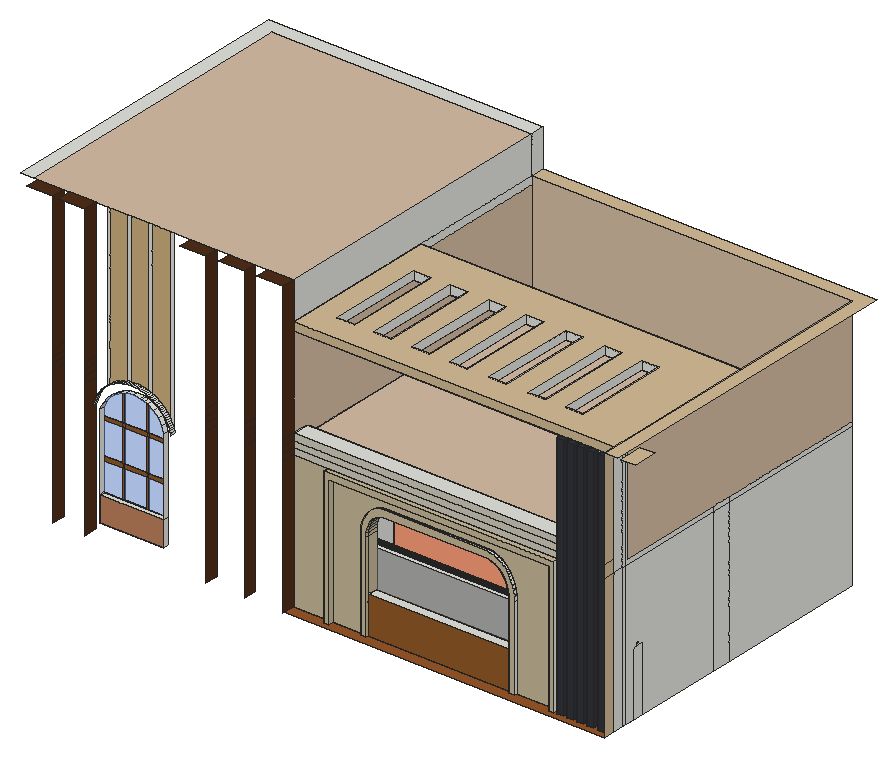
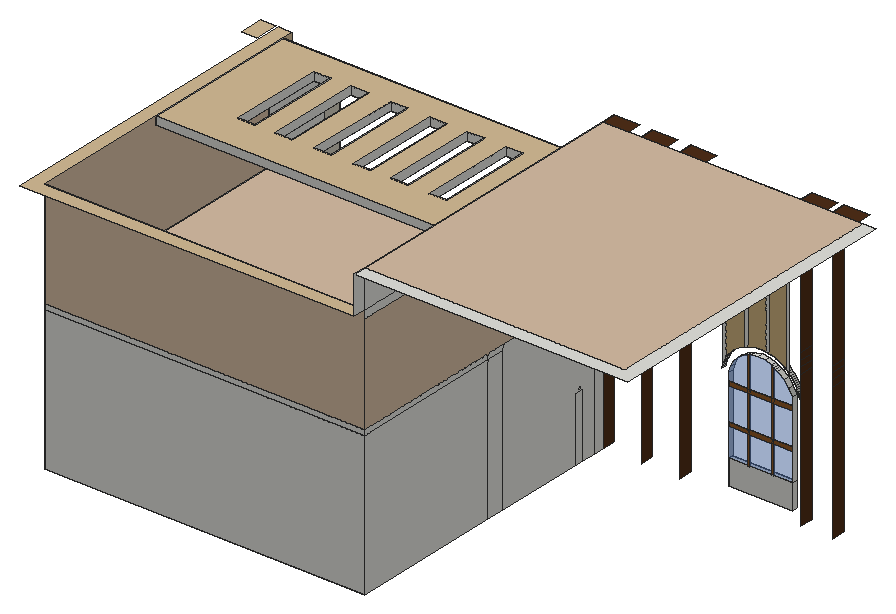
# SketchUp Ruby script. Lengths in inches.
U = 1.inch
M = Sketchup.active_model
def pt(a) = Geom::Point3d.new(a.map { |v| v * U })
def face(e, loops, mat)
  f = e.add_face(loops[0].map { |a| pt(a) })
  loops[1..].each { |l| e.add_face(l.map { |a| pt(a) }).erase! }
  f.material = f.back_material = mat if mat
  f
end
# faces: each face lists its corners as indices into pts; further lists are holes
def faces(e, pts, list, mat = nil) = list.each { |f| face(e, (f[0].is_a?(Array) ? f : [f]).map { |l| l.map { |i| pts[i] } }, mat) }
# xy, xz, yz: faces in a plane at the given z, y or x. An outline is a flat list of corners, or four numbers for a rectangle; further outlines are holes
def ring(l) = l.size == 4 ? [[l[0], l[1]], [l[2], l[1]], [l[2], l[3]], [l[0], l[3]]] : l.each_slice(2).to_a
def flat(e, list, mat, &to3) = list.each { |f| face(e, (f[0].is_a?(Array) ? f : [f]).map { |l| ring(l).map { |u, v| to3.(u, v) } }, mat) }
def xy(e, z, list, mat = nil) = flat(e, list, mat) { |x, y| [x, y, z] }
def xz(e, y, list, mat = nil) = flat(e, list, mat) { |x, z| [x, y, z] }
def yz(e, x, list, mat = nil) = flat(e, list, mat) { |y, z| [x, y, z] }
def lines(e, pts, list) = list.each { |a, b| e.add_line(pt(pts[a]), pt(pts[b])) }
# prism: a flat outline (further loops are holes) pulled along v
def prism(e, loops, v, mat = nil)
  f = face(e, loops, mat); d = Geom::Vector3d.new(v.map { |x| x * U })
  f.pushpull(f.normal.samedirection?(d) ? d.length : -d.length)
end
def box(e, o, s, mat = nil) = prism(e, [[o, [o[0] + s[0], o[1], o[2]], [o[0] + s[0], o[1] + s[1], o[2]], [o[0], o[1] + s[1], o[2]]]], [0, 0, s[2]], mat)
def at(x, y, z, deg = 0) = Geom::Transformation.translation(pt([x, y, z])) * Geom::Transformation.rotation(ORIGIN, Z_AXIS, deg.degrees)
def axes(o, x, y, z) = Geom::Transformation.new([*x, 0, *y, 0, *z, 0, *pt(o).to_a, 1])
def part(name) = M.definitions.add(name)
# library, detail: a bought-in or finely detailed component or shape, given as its bounding box
def library(name, o, s) = part(name).tap { |d| box(d.entities, o, s) }
def detail(e, o, s) = box(e.add_group.entities, o, s)
def put(e, d, t, mat = nil) = e.add_instance(d, t).tap { |i| i.material = mat if mat }
def group(e, t, mat = nil) = e.add_group.tap { |g| g.transformation = t; g.material = mat if mat }.entities
root = M.entities
M.materials.add("[0026_LightSalmon]").color = [255, 160, 122]
M.materials.add("[Blinds Cloth Horizontal]").color = [192, 163, 85]
M.materials.add("[Formica Beige]").color = [211, 187, 149]
M.materials.add("[Formica Graystone]").color = [209, 204, 189]
M.materials.add("[Formica Laminate Dark]").color = [50, 53, 60]
M.materials.add("[Formica Laminate Light]").color = [213, 189, 164]
M.materials.add("[Quartz Light Brown]").color = [199, 184, 152]
M.materials.add("[Translucent Glass Blue]").color = [100, 149, 237]
M.materials["[Translucent Glass Blue]"].alpha = 0.5
M.materials.add("[Translucent Glass Gray]").color = [128, 128, 128]
M.materials["[Translucent Glass Gray]"].alpha = 0.5
M.materials.add("[Wood Board Cork]").color = [215, 201, 115]
M.materials.add("[Wood Cherry Original]").color = [152, 86, 42]
M.materials.add("[Wood Floor Light]").color = [204, 176, 127]
M.materials.add("[Wood Floor Parquet]").color = [145, 89, 39]
M.materials.add("[Wood Lumber ButtJoined]").color = [164, 152, 112]
M.materials.add("[Wood Veneer 01]").color = [79, 46, 24]
M.materials.add("[Wood Veneer 02]").color = [190, 128, 91]
xy(root,384.375,[[396.28,197.36,402.37,203.79],[656.81,197.36,662.9,203.79],[665.86,197.92,673.64,203.79],[677.3,197.92,685.08,203.79],[688.86,197.92,696.64,203.79],
  [700.67,197.92,708.46,203.79],[713.49,197.92,721.27,203.79],[436.36,200.73,443.05,203.79],[608.17,200.73,614.86,203.79],[356.6875,203.79,443.05,215.49],
  [443.05,203.79,608.17,215.49],[608.17,203.79,727.17,215.49],[356.6875,215.49,727.17,232.67],[356.6875,232.67,727.17,244.16],[356.6875,244.16,727.17,348.07],
  [356.6875,348.07,727.17,370.07],[356.6875,370.07,727.17,548.03]])
xy(root,384.375,[[356.6875,190.11,727.17,190.11,727.17,203.79,721.27,203.79,721.27,197.92,713.49,197.92,713.49,203.79,708.46,203.79,708.46,197.92,700.67,197.92,700.67,203.79,696.64,203.79,696.64,197.92,688.86,197.92,688.86,203.79,685.08,203.79,685.08,197.92,677.3,197.92,677.3,203.79,673.64,203.79,673.64,197.92,665.86,197.92,665.86,203.79,662.9,203.79,662.9,197.36,656.81,197.36,656.81,203.79,614.86,203.79,614.86,200.73,608.17,200.73,608.17,203.79,443.05,203.79,443.05,200.73,436.36,200.73,436.36,203.79,402.37,203.79,402.37,197.36,396.28,197.36,396.28,203.79,356.6875,203.79]],"[Wood Cherry Original]")
xy(root,397.07,[[137.48,197.92,211.51,203.79]])
xy(root,425.68,[[137.48,197.92,211.51,203.79]])
xy(root,427.25,[[443.05,203.79,608.17,215.49]])
xy(root,436.87,[[372.34,348.07,438.53,355.26]])
xy(root,458.75,[[356.6875,232.67,727.17,244.16]])
xy(root,514.98,[[463.23,200.73,582.11,203.79],[463.23,203.79,582.11,215.49]])
xy(root,519.81,[[372.34,348.07,438.53,355.26]])
xy(root,522.81,[[462.98,200.73,582.35,203.79]],"[Quartz Light Brown]")
xy(root,534.39,[[402.37,197.36,656.81,203.79]])
xy(root,541.34,[[396.28,197.36,662.9,203.79]],"[Quartz Light Brown]")
xy(root,549,[[356.6875,348.07,727.17,370.07],[356.6875,370.07,727.17,548.03]])
xy(root,555.125,[[356.6875,223.7,727.17,548.03]],"[Formica Laminate Light]")
xy(root,563.875,[[356.6875,203.79,662.9,223.7]])
xy(root,670.25,[[[356.6875,203.79,356.6875,387.77,727.17,387.77,727.17,223.7,662.9,223.7,662.9,203.79],[382.94,233.99,402.82,344.43],[425.38,233.99,445.26,344.43],[469.76,233.99,489.63,344.43],[513.32,233.99,533.19,344.43],[558.69,233.99,578.57,344.43],[604.07,233.99,623.94,344.43],[647.13,233.99,667.01,344.43]]],"[Formica Beige]")
xy(root,670.25,[[665.86,197.92,673.64,203.79],[677.3,197.92,685.08,203.79],[688.86,197.92,696.64,203.79],[700.67,197.92,708.46,203.79],[713.49,197.92,721.27,203.79]],"[Formica Laminate Dark]")
xy(root,679.64,[[727.17,190.11,742.93,190.11,742.93,563.79,356.6875,563.79,356.6875,548.03,727.17,548.03],[746.31,190.11,763.24,218.11],[[356.6875,203.79,727.17,387.77],[382.94,233.99,402.82,344.43],[425.38,233.99,445.26,344.43],[469.76,233.99,489.63,344.43],[513.32,233.99,533.19,344.43],[558.69,233.99,578.57,344.43],[604.07,233.99,623.94,344.43],[647.13,233.99,667.01,344.43]]],"[Formica Beige]")
xy(root,723.1875,[[40.4375,203.79,56.2,203.79,56.2,548.03,356.6875,548.03,356.6875,563.79,40.4375,563.79]])
xy(root,723.1875,[[56.2,203.79,356.6875,548.03]],"[Formica Laminate Light]")
xy(root,723.1875,[[61.07,188.11,91,203.79],[98.07,188.11,128,203.79],[238.01,188.11,267.9375,203.79],[282.39,188.11,312.3125,203.79],[326.76,188.11,356.6875,203.79]],"[Wood Veneer 01]")
xz(root,197.36,[[396.28,384.375,402.37,384.375,402.37,534.39,656.81,534.39,656.81,384.375,662.9,384.375,662.9,541.34,396.28,541.34]],"[Quartz Light Brown]")
xz(root,197.92,[[665.86,384.375,673.64,670.25],[677.3,384.375,685.08,670.25],[688.86,384.375,696.64,670.25],[700.67,384.375,708.46,670.25],[713.49,384.375,721.27,670.25]],"[Formica Laminate Dark]")
xz(root,197.92,[[137.48,397.07,211.51,425.68]],"[Wood Veneer 02]")
xz(root,200.73,[[436.36,384.375,443.05,384.375,443.05,488.3125,443.24,492.08,443.78,495.56,444.66,498.89,445.86,502.03,447.36,504.91,449.12,507.5,451.1,509.73,453.26,511.6,455.57,513.0625,457.99,514.12,460.47,514.75,463.23,514.98,582.11,514.98,585.64,514.6875,588.875,513.86,592.02,512.48,595.02,510.58,597.82,508.17,600.38,505.28,602.65,501.95,604.57,498.24,606.12,494.22,607.25,489.94,607.93,485.5,608.17,480.74,608.17,384.375,614.86,384.375,614.86,480.97,614.58,486.43,613.75,491.8,612.39,496.98,610.51,501.89,608.14,506.4375,605.34,510.55,602.14,514.16,598.61,517.2,594.79,519.625,590.77,521.38,586.6,522.45,582.35,522.81,462.98,522.81,459.51,522.51,456.09,521.64,452.8,520.2,449.67,518.22,446.78,515.73,444.16,512.77,441.86,509.4,439.93,505.68,438.39,501.66,437.27,497.41,436.59,493.02,436.36,488.54]],"[Quartz Light Brown]")
xz(root,203.79,[[396.28,384.375,396.28,541.34,662.9,541.34,662.9,384.375,656.81,384.375,656.81,534.39,402.37,534.39,402.37,384.375],[436.36,384.375,436.36,488.54,436.59,493.02,437.27,497.41,438.39,501.66,439.93,505.68,441.86,509.4,444.16,512.77,446.78,515.73,449.67,518.22,452.8,520.2,456.09,521.64,459.51,522.51,462.98,522.81,582.35,522.81,586.6,522.45,590.77,521.38,594.79,519.625,598.61,517.2,602.14,514.16,605.34,510.55,608.14,506.4375,610.51,501.89,612.39,496.98,613.75,491.8,614.58,486.43,614.86,480.97,614.86,384.375,608.17,384.375,608.17,480.74,607.93,485.5,607.25,489.94,606.12,494.22,604.57,498.24,602.65,501.95,600.38,505.28,597.82,508.17,595.02,510.58,592.02,512.48,588.875,513.86,585.64,514.6875,582.11,514.98,463.23,514.98,460.47,514.75,457.99,514.12,455.57,513.0625,453.26,511.6,451.1,509.73,449.12,507.5,447.36,504.91,445.86,502.03,444.66,498.89,443.78,495.56,443.24,492.08,443.05,488.3125,443.05,384.375],[665.86,384.375,673.64,670.25],[673.64,384.375,677.3,670.25],[677.3,384.375,685.08,670.25],
  [685.08,384.375,688.86,670.25],[688.86,384.375,696.64,670.25],[696.64,384.375,700.67,670.25],[700.67,384.375,708.46,670.25],[708.46,384.375,713.49,670.25],
  [713.49,384.375,721.27,670.25],[721.27,384.375,727.17,670.25],[137.48,397.07,211.51,425.68],[218.4,519.9,218.4,723.1875,215.12,723.1875,215.12,527.48,216.07,525.64,216.93,523.77,217.71,521.85],[141.18,537.45,142.64,538.91,144.17,540.3,144.17,723.1875,141.18,723.1875],
  [192.6,547.93,192.6,723.1875,188.73,723.1875,188.73,549.38,190.68,548.7],[164.25,550.47,166.27,550.89,168.3125,551.21,168.3125,723.1875,164.25,723.1875]])
xz(root,203.79,[[356.6875,670.25,727.17,679.64]],"[Formica Beige]")
xz(root,203.79,[[662.9,384.375,665.86,670.25],[356.6875,541.34,662.9,549],[356.6875,549,662.9,556.4375],[356.6875,556.4375,662.9,563.875]],"[Formica Graystone]")
xz(root,203.79,[[356.6875,384.375,396.28,541.34],[402.37,384.375,436.36,384.375,436.36,488.54,436.59,493.02,437.27,497.41,438.39,501.66,439.93,505.68,441.86,509.4,444.16,512.77,446.78,515.73,449.67,518.22,452.8,520.2,456.09,521.64,459.51,522.51,462.98,522.81,582.35,522.81,586.6,522.45,590.77,521.38,594.79,519.625,598.61,517.2,602.14,514.16,605.34,510.55,608.14,506.4375,610.51,501.89,612.39,496.98,613.75,491.8,614.58,486.43,614.86,480.97,614.86,384.375,656.81,384.375,656.81,534.39,402.37,534.39]],"[Quartz Light Brown]")
xz(root,203.79,[[137.48,425.68,158.65,458.55],[161.03,425.68,186.27,458.55],[188.66,425.68,211.51,458.55],[137.48,463.21,158.65,500.75],[161.03,463.21,186.27,500.75],
  [188.66,463.21,211.51,500.75],[137.48,505.34,158.65,505.34,158.65,538.17,156.35,536.79,153.96,535.3,146.84,529.54,141.18,522.34,137.48,514.54],[161.03,505.34,186.27,505.34,186.27,541.26,184.83,541.79,176.79,542.85,168.71,542.1,161,539.58,161.03,533.51],[188.66,505.34,211.51,505.34,211.51,514.54,209.09,521.8,204.875,528.73,199.23,534.55,192.4375,538.98,188.66,540.38]],"[Translucent Glass Blue]")
xz(root,203.79,[[215.12,527.48,215.12,723.1875,192.6,723.1875,192.6,547.93,194.48,547.08,196.33,546.15,198.125,545.13,199.88,544.04,201.58,542.87,203.23,541.62,204.82,540.3,206.35,538.91,207.8125,537.45,209.21,535.93,210.54,534.35,211.8,532.71,212.99,531.02,214.09,529.27],[144.17,540.3,145.76,541.62,147.41,542.87,149.11,544.04,150.87,545.13,152.66,546.15,154.51,547.08,156.39,547.93,158.3125,548.7,160.26,549.38,162.24,549.97,164.25,550.47,164.25,723.1875,144.17,723.1875],[188.73,549.38,188.73,723.1875,168.3125,723.1875,168.3125,551.21,170.37,551.44,172.43,551.58,174.5,551.625,176.5625,551.58,178.625,551.44,180.68,551.21,182.72,550.89,184.74,550.47,186.75,549.97]],"[Wood Floor Light]")
xz(root,203.79,[[443.05,384.375,608.17,427.25],[158.65,425.68,161.03,458.55],[186.27,425.68,188.66,458.55],[137.48,458.55,158.65,463.21],[158.65,458.55,161.03,463.21],
  [161.03,458.55,186.27,463.21],[186.27,458.55,188.66,463.21],[188.66,458.55,211.51,463.21],[158.65,463.21,161.03,500.75],[186.27,463.21,188.66,500.75],
  [137.48,500.75,158.65,505.34],[158.65,500.75,161.03,505.34],[161.03,500.75,186.27,505.34],[186.27,500.75,188.66,505.34],[188.66,500.75,211.51,505.34],
  [158.65,505.34,161.03,505.34,161.03,533.51,161,539.58,158.65,538.17],[186.27,505.34,188.66,505.34,188.66,540.38,186.27,541.26]],"[Wood Floor Parquet]")
xz(root,215.49,[[443.05,384.375,608.17,427.25]])
xz(root,223.7,[[356.6875,555.125,662.9,563.875],[662.9,555.125,727.17,670.25]])
xz(root,232.67,[[356.6875,384.375,727.17,458.75]],"[Translucent Glass Gray]")
xz(root,233.99,[[382.94,670.25,402.82,679.64],[425.38,670.25,445.26,679.64],[469.76,670.25,489.63,679.64],[513.32,670.25,533.19,679.64],[558.69,670.25,578.57,679.64],
  [604.07,670.25,623.94,679.64],[647.13,670.25,667.01,679.64]])
xz(root,244.16,[[356.6875,384.375,727.17,458.75]])
xz(root,344.43,[[382.94,670.25,402.82,679.64],[425.38,670.25,445.26,679.64],[469.76,670.25,489.63,679.64],[513.32,670.25,533.19,679.64],[558.69,670.25,578.57,679.64],
  [604.07,670.25,623.94,679.64],[647.13,670.25,667.01,679.64]])
xz(root,348.07,[[[356.6875,384.375,630.64,384.375,630.64,526.3125,701.89,526.3125,701.89,384.375,727.17,384.375,727.17,549,356.6875,549],[473.14,434.83,573.76,527.39],[372.34,436.87,438.53,519.81]]],"[0026_LightSalmon]")
xz(root,348.07,[[478.96,440.65,520.59,521.5625],[526.38,440.65,567.9375,521.5625]],"[Blinds Cloth Horizontal]")
xz(root,348.07,[[636.07,469.29,691.81,520.89,687.15,520.89,663.14,499.1,661.61,497.71,636.07,474.53],[661.61,497.71,663.14,499.1,653.11,520.89,649.25,520.89]],"[Wood Board Cork]")
xz(root,348.07,[[[636.07,389.8,696.47,389.8,696.47,520.89,691.81,520.89,636.07,469.29],[640.62,439.3125,644.62,462.125]],[636.07,474.53,661.61,497.71,649.25,520.89,636.07,520.89],[663.14,499.1,687.15,520.89,653.11,520.89]],"[Wood Floor Light]")
xz(root,348.07,[[[630.64,384.375,701.89,526.3125],[636.07,389.8,696.47,520.89]],[[473.14,434.83,573.76,527.39],[478.96,440.65,567.9375,521.5625]],[520.59,440.65,526.38,521.5625]],"[Wood Floor Parquet]")
xz(root,348.07,[[640.62,439.3125,644.62,462.125]],"[Wood Lumber ButtJoined]")
xz(root,355.26,[[377.09,441.62,401.32,515.0625],[406.17,441.62,433.78,515.0625]],"[Blinds Cloth Horizontal]")
xz(root,355.26,[[[372.34,436.87,438.53,519.81],[377.09,441.62,433.78,515.0625]],[401.32,441.62,406.17,515.0625]],"[Wood Floor Parquet]")
xz(root,370.07,[[356.6875,384.375,727.17,549]])
xz(root,387.77,[[356.6875,670.25,727.17,679.64]])
xz(root,548.03,[[356.6875,384.375,727.17,549],[356.6875,549,727.17,555.125]])
xz(root,548.03,[[356.6875,555.125,727.17,679.64]],"[Formica Laminate Light]")
yz(root,91,[[188.11,384.375,203.79,541.34],[188.11,541.34,203.79,549],[188.11,549,203.79,556.4375],[188.11,556.4375,203.79,563.875],[188.11,563.875,203.79,723.1875]],"[Wood Veneer 01]")
yz(root,128,[[188.11,384.375,203.79,541.34],[188.11,541.34,203.79,549],[188.11,549,203.79,556.4375],[188.11,556.4375,203.79,563.875],[188.11,563.875,203.79,723.1875]],"[Wood Veneer 01]")
yz(root,137.48,[[197.92,397.07,203.79,425.68],[197.92,425.68,203.79,514.54]])
yz(root,211.51,[[197.92,397.07,203.79,425.68],[197.92,425.68,203.79,514.54]])
yz(root,267.9375,[[188.11,384.375,203.79,541.34],[188.11,541.34,203.79,549],[188.11,549,203.79,556.4375],[188.11,556.4375,203.79,563.875],[188.11,563.875,203.79,723.1875]],"[Wood Veneer 01]")
yz(root,312.3125,[[188.11,384.375,203.79,541.34],[188.11,541.34,203.79,549],[188.11,549,203.79,556.4375],[188.11,556.4375,203.79,563.875],[188.11,563.875,203.79,723.1875]],"[Wood Veneer 01]")
yz(root,356.6875,[[203.79,384.375,215.49,563.875],[[215.49,384.375,232.67,384.375,232.67,458.75,244.16,458.75,244.16,384.375,348.07,384.375,348.07,555.125,223.7,555.125,223.7,563.875,215.49,563.875],[237.55,459.44,236.99,459.51,236.46,459.73,236.01,460.08,235.66,460.53,235.44,461.06,235.37,461.62,235.44,462.1875,235.66,462.72,236.01,463.17,236.46,463.52,236.99,463.74,237.55,463.81,238.12,463.74,238.65,463.52,239.1,463.17,239.45,462.72,239.67,462.1875,239.74,461.62,239.67,461.06,239.45,460.53,239.1,460.08,238.65,459.73,238.12,459.51]],[232.67,384.375,244.16,458.75],[348.07,384.375,370.07,549],[370.07,384.375,548.03,549],
  [237.55,459.44,236.99,459.51,236.46,459.73,236.01,460.08,235.66,460.53,235.44,461.06,235.37,461.62,235.44,462.1875,235.66,462.72,236.01,463.17,236.46,463.52,236.99,463.74,237.55,463.81,238.12,463.74,238.65,463.52,239.1,463.17,239.45,462.72,239.67,462.1875,239.74,461.62,239.67,461.06,239.45,460.53,239.1,460.08,238.65,459.73,238.12,459.51],[348.07,549,370.07,555.125],[370.07,549,548.03,555.125],[203.79,670.25,387.77,679.64],[387.77,670.25,548.03,679.64],
  [203.79,679.64,548.03,723.1875],[548.03,679.64,563.79,723.1875]])
yz(root,356.6875,[[223.7,555.125,548.03,555.125,548.03,670.25,203.79,670.25,203.79,563.875,223.7,563.875]],"[Formica Laminate Light]")
yz(root,356.6875,[[188.11,384.375,203.79,541.34],[188.11,541.34,203.79,549],[188.11,549,203.79,556.4375],[188.11,556.4375,203.79,563.875],[188.11,563.875,203.79,723.1875]],"[Wood Veneer 01]")
yz(root,372.34,[[348.07,436.87,355.26,519.81]])
yz(root,382.94,[[233.99,670.25,344.43,679.64]])
yz(root,396.28,[[197.36,384.375,203.79,541.34]],"[Quartz Light Brown]")
yz(root,402.37,[[197.36,384.375,203.79,534.39]],"[Quartz Light Brown]")
yz(root,402.82,[[233.99,670.25,344.43,679.64]])
yz(root,425.38,[[233.99,670.25,344.43,679.64]])
yz(root,436.36,[[200.73,384.375,203.79,488.54]],"[Quartz Light Brown]")
yz(root,438.53,[[348.07,436.87,355.26,519.81]])
yz(root,443.05,[[203.79,384.375,215.49,427.25]])
yz(root,443.05,[[200.73,384.375,203.79,488.3125],[203.79,427.25,215.49,488.3125]],"[Quartz Light Brown]")
yz(root,445.26,[[233.99,670.25,344.43,679.64]])
yz(root,469.76,[[233.99,670.25,344.43,679.64]])
yz(root,489.63,[[233.99,670.25,344.43,679.64]])
yz(root,513.32,[[233.99,670.25,344.43,679.64]])
yz(root,533.19,[[233.99,670.25,344.43,679.64]])
yz(root,558.69,[[233.99,670.25,344.43,679.64]])
yz(root,578.57,[[233.99,670.25,344.43,679.64]])
yz(root,604.07,[[233.99,670.25,344.43,679.64]])
yz(root,608.17,[[203.79,384.375,215.49,427.25]])
yz(root,608.17,[[200.73,384.375,203.79,480.74],[203.79,427.25,215.49,480.74]],"[Quartz Light Brown]")
yz(root,614.86,[[200.73,384.375,203.79,480.97]])
yz(root,623.94,[[233.99,670.25,344.43,679.64]])
yz(root,647.13,[[233.99,670.25,344.43,679.64]])
yz(root,656.81,[[197.36,384.375,203.79,534.39]],"[Quartz Light Brown]")
yz(root,662.9,[[197.36,384.375,203.79,541.34]])
yz(root,662.9,[[203.79,563.875,223.7,670.25]],"[Formica Graystone]")
yz(root,665.86,[[197.92,384.375,203.79,670.25]],"[Formica Laminate Dark]")
yz(root,667.01,[[233.99,670.25,344.43,679.64]])
yz(root,673.64,[[197.92,384.375,203.79,670.25]],"[Formica Laminate Dark]")
yz(root,677.3,[[197.92,384.375,203.79,670.25]],"[Formica Laminate Dark]")
yz(root,685.08,[[197.92,384.375,203.79,670.25]],"[Formica Laminate Dark]")
yz(root,688.86,[[197.92,384.375,203.79,670.25]],"[Formica Laminate Dark]")
yz(root,696.64,[[197.92,384.375,203.79,670.25]],"[Formica Laminate Dark]")
yz(root,700.67,[[197.92,384.375,203.79,670.25]],"[Formica Laminate Dark]")
yz(root,708.46,[[197.92,384.375,203.79,670.25]],"[Formica Laminate Dark]")
yz(root,713.49,[[197.92,384.375,203.79,670.25]],"[Formica Laminate Dark]")
yz(root,721.27,[[197.92,384.375,203.79,670.25]],"[Formica Laminate Dark]")
yz(root,727.17,[[203.79,384.375,215.49,549],[215.49,384.375,219.56,549],[[219.56,384.375,219.56,549,348.07,549,348.07,384.375,244.16,384.375,244.16,458.75,232.67,458.75,232.67,384.375],[237.55,459.44,238.12,459.51,238.65,459.73,239.1,460.08,239.45,460.53,239.67,461.06,239.74,461.62,239.67,462.1875,239.45,462.72,239.1,463.17,238.65,463.52,238.12,463.74,237.55,463.81,236.99,463.74,236.46,463.52,236.01,463.17,235.66,462.72,235.44,462.1875,235.37,461.62,235.44,461.06,235.66,460.53,236.01,460.08,236.46,459.73,236.99,459.51]],[232.67,384.375,244.16,458.75],[348.07,384.375,370.07,549],
  [370.07,384.375,548.03,549],[203.79,549,215.49,670.25],[215.49,549,219.56,670.25],[219.56,549,348.07,549,348.07,555.125,223.7,555.125,223.7,670.25,219.56,670.25],[348.07,549,370.07,555.125],
  [370.07,549,548.03,555.125],[203.79,670.25,215.49,679.64],[215.49,670.25,219.56,679.64],[219.56,670.25,387.77,679.64]])
yz(root,727.17,[[190.11,384.375,203.79,549],[190.11,549,203.79,563.875],[190.11,563.875,203.79,679.64]],"[Formica Beige]")
yz(root,727.17,[[223.7,555.125,223.7,670.25,387.77,670.25,387.77,679.64,548.03,679.64,548.03,555.125]],"[Formica Laminate Light]")
p = [[356.6875,236.99,459.51],[356.6875,237.55,459.44],[727.17,237.55,459.44],[727.17,236.99,459.51],[356.6875,238.12,459.51],[727.17,238.12,459.51],
  [356.6875,236.46,459.73],[727.17,236.46,459.73],[356.6875,238.65,459.73],[727.17,238.65,459.73],[356.6875,236.01,460.08],[727.17,236.01,460.08],
  [356.6875,239.1,460.08],[727.17,239.1,460.08],[356.6875,235.66,460.53],[727.17,235.66,460.53],[356.6875,239.45,460.53],[727.17,239.45,460.53],
  [356.6875,235.44,461.06],[727.17,235.44,461.06],[356.6875,239.67,461.06],[727.17,239.67,461.06],[356.6875,235.37,461.62],[727.17,235.37,461.62],
  [356.6875,239.74,461.62],[727.17,239.74,461.62],[356.6875,235.44,462.1875],[727.17,235.44,462.1875],[356.6875,239.67,462.1875],[727.17,239.67,462.1875],
  [356.6875,235.66,462.72],[727.17,235.66,462.72],[356.6875,239.45,462.72],[727.17,239.45,462.72],[356.6875,236.01,463.17],[727.17,236.01,463.17],
  [356.6875,239.1,463.17],[727.17,239.1,463.17],[356.6875,236.46,463.52],[727.17,236.46,463.52],[356.6875,238.65,463.52],[727.17,238.65,463.52],
  [356.6875,236.99,463.74],[727.17,236.99,463.74],[356.6875,238.12,463.74],[727.17,238.12,463.74],[356.6875,237.55,463.81],[727.17,237.55,463.81],
  [607.93,203.79,485.5],[608.17,203.79,480.74],[608.17,200.73,480.74],[607.93,200.73,485.5],[607.93,215.49,485.5],[608.17,215.49,480.74],
  [614.86,203.79,480.97],[614.58,203.79,486.43],[614.58,200.73,486.43],[614.86,200.73,480.97],[607.25,203.79,489.94],[607.25,200.73,489.94],
  [607.25,215.49,489.94],[613.75,203.79,491.8],[613.75,200.73,491.8],[443.05,203.79,488.3125],[443.24,203.79,492.08],[443.24,200.73,492.08],
  [443.05,200.73,488.3125],[443.05,215.49,488.3125],[443.24,215.49,492.08],[436.59,203.79,493.02],[436.36,203.79,488.54],[436.36,200.73,488.54],
  [436.59,200.73,493.02],[606.12,203.79,494.22],[606.12,200.73,494.22],[606.12,215.49,494.22],[612.39,203.79,496.98],[612.39,200.73,496.98],
  [443.78,203.79,495.56],[443.78,200.73,495.56],[443.78,215.49,495.56],[437.27,203.79,497.41],[437.27,200.73,497.41],[604.57,203.79,498.24],
  [604.57,200.73,498.24],[604.57,215.49,498.24],[444.66,203.79,498.89],[444.66,200.73,498.89],[444.66,215.49,498.89],[610.51,203.79,501.89],
  [610.51,200.73,501.89],[438.39,203.79,501.66],[438.39,200.73,501.66],[602.65,203.79,501.95],[602.65,200.73,501.95],[602.65,215.49,501.95],
  [445.86,203.79,502.03],[445.86,200.73,502.03],[445.86,215.49,502.03],[439.93,203.79,505.68],[439.93,200.73,505.68],[608.14,203.79,506.4375],
  [608.14,200.73,506.4375],[447.36,203.79,504.91],[447.36,200.73,504.91],[600.38,203.79,505.28],[600.38,200.73,505.28],[447.36,215.49,504.91],
  [600.38,215.49,505.28],[449.12,203.79,507.5],[449.12,200.73,507.5],[449.12,215.49,507.5],[597.82,203.79,508.17],[597.82,200.73,508.17],
  [597.82,215.49,508.17],[441.86,203.79,509.4],[441.86,200.73,509.4],[605.34,203.79,510.55],[605.34,200.73,510.55],[451.1,203.79,509.73],
  [451.1,200.73,509.73],[451.1,215.49,509.73],[595.02,203.79,510.58],[595.02,200.73,510.58],[595.02,215.49,510.58],[444.16,203.79,512.77],
  [444.16,200.73,512.77],[453.26,203.79,511.6],[453.26,200.73,511.6],[453.26,215.49,511.6],[592.02,203.79,512.48],[592.02,200.73,512.48],
  [602.14,203.79,514.16],[602.14,200.73,514.16],[592.02,215.49,512.48],[455.57,203.79,513.0625],[455.57,200.73,513.0625],[455.57,215.49,513.0625],
  [588.875,203.79,513.86],[588.875,200.73,513.86],[588.875,215.49,513.86],[446.78,203.79,515.73],[446.78,200.73,515.73],[457.99,203.79,514.12],
  [457.99,200.73,514.12],[457.99,215.49,514.12],[585.64,203.79,514.6875],[585.64,200.73,514.6875],[585.64,215.49,514.6875],[460.47,203.79,514.75],
  [460.47,200.73,514.75],[460.47,215.49,514.75],[598.61,203.79,517.2],[598.61,200.73,517.2],[137.48,203.79,514.54],[141.18,203.79,522.34],
  [141.18,197.92,522.34],[137.48,197.92,514.54],[209.09,203.79,521.8],[211.51,203.79,514.54],[211.51,197.92,514.54],[209.09,197.92,521.8],
  [582.11,203.79,514.98],[582.11,200.73,514.98],[582.11,215.49,514.98],[463.23,203.79,514.98],[463.23,200.73,514.98],[463.23,215.49,514.98],
  [449.67,203.79,518.22],[449.67,200.73,518.22],[129.98,203.79,517.93],[129.46,203.79,515.93],[129.46,197.92,515.93],[129.98,197.92,517.93],
  [219.53,203.79,515.93],[219.01,203.79,517.93],[219.01,197.92,517.93],[219.53,197.92,515.93],[594.79,203.79,519.625],[594.79,200.73,519.625],
  [130.59,203.79,519.9],[130.59,197.92,519.9],[218.4,203.79,519.9],[218.4,197.92,519.9],[452.8,203.79,520.2],[452.8,200.73,520.2],
  [590.77,203.79,521.38],[590.77,200.73,521.38],[131.28,203.79,521.85],[131.28,197.92,521.85],[217.71,203.79,521.85],[217.71,197.92,521.85],
  [456.09,203.79,521.64],[456.09,200.73,521.64],[586.6,203.79,522.45],[586.6,200.73,522.45],[459.51,203.79,522.51],[459.51,200.73,522.51],
  [204.875,203.79,528.73],[204.875,197.92,528.73],[132.06,203.79,523.77],[132.06,197.92,523.77],[216.93,203.79,523.77],[216.93,197.92,523.77],
  [146.84,203.79,529.54],[146.84,197.92,529.54],[462.98,203.79,522.81],[462.98,200.73,522.81],[582.35,203.79,522.81],[582.35,200.73,522.81],
  [132.92,203.79,525.64],[132.92,197.92,525.64],[216.07,203.79,525.64],[216.07,197.92,525.64],[133.87,203.79,527.48],[133.87,197.92,527.48],
  [215.12,203.79,527.48],[215.12,197.92,527.48],[134.9,203.79,529.27],[134.9,197.92,529.27],[214.09,203.79,529.27],[214.09,197.92,529.27],
  [199.23,203.79,534.55],[199.23,197.92,534.55],[136,203.79,531.02],[136,197.92,531.02],[212.99,203.79,531.02],[212.99,197.92,531.02],
  [153.96,203.79,535.3],[153.96,197.92,535.3],[137.1875,203.79,532.71],[137.1875,197.92,532.71],[211.8,203.79,532.71],[211.8,197.92,532.71],
  [138.45,203.79,534.35],[138.45,197.92,534.35],[210.54,203.79,534.35],[210.54,197.92,534.35],[139.78,203.79,535.93],[139.78,197.92,535.93],
  [209.21,203.79,535.93],[209.21,197.92,535.93],[192.4375,203.79,538.98],[192.4375,197.92,538.98],[156.35,203.79,536.79],[156.35,197.92,536.79],
  [141.18,203.79,537.45],[141.18,197.92,537.45],[207.8125,203.79,537.45],[207.8125,197.92,537.45],[158.65,203.79,538.17],[158.65,197.92,538.17],
  [142.64,203.79,538.91],[142.64,197.92,538.91],[206.35,203.79,538.91],[206.35,197.92,538.91],[161,203.79,539.58],[161,197.92,539.58],
  [144.17,203.79,540.3],[144.17,197.92,540.3],[204.82,203.79,540.3],[204.82,197.92,540.3],[188.66,203.79,540.38],[188.66,197.92,540.38],
  [168.71,203.79,542.1],[168.71,197.92,542.1],[145.76,203.79,541.62],[145.76,197.92,541.62],[203.23,203.79,541.62],[203.23,197.92,541.62],
  [186.27,203.79,541.26],[186.27,197.92,541.26],[184.83,203.79,541.79],[184.83,197.92,541.79],[147.41,203.79,542.87],[147.41,197.92,542.87],
  [201.58,203.79,542.87],[201.58,197.92,542.87],[176.79,203.79,542.85],[176.79,197.92,542.85],[149.11,203.79,544.04],[149.11,197.92,544.04],
  [199.88,203.79,544.04],[199.88,197.92,544.04],[150.87,203.79,545.13],[150.87,197.92,545.13],[198.125,203.79,545.13],[198.125,197.92,545.13],
  [152.66,203.79,546.15],[152.66,197.92,546.15],[196.33,203.79,546.15],[196.33,197.92,546.15],[154.51,203.79,547.08],[154.51,197.92,547.08],
  [194.48,203.79,547.08],[194.48,197.92,547.08],[156.39,203.79,547.93],[156.39,197.92,547.93],[192.6,203.79,547.93],[192.6,197.92,547.93],
  [158.3125,203.79,548.7],[158.3125,197.92,548.7],[190.68,203.79,548.7],[190.68,197.92,548.7],[160.26,203.79,549.38],[160.26,197.92,549.38],
  [188.73,203.79,549.38],[188.73,197.92,549.38],[162.24,203.79,549.97],[162.24,197.92,549.97],[186.75,203.79,549.97],[186.75,197.92,549.97],
  [164.25,203.79,550.47],[164.25,197.92,550.47],[184.74,203.79,550.47],[184.74,197.92,550.47],[166.27,203.79,550.89],[166.27,197.92,550.89],
  [182.72,203.79,550.89],[182.72,197.92,550.89],[168.3125,203.79,551.21],[168.3125,197.92,551.21],[180.68,203.79,551.21],[180.68,197.92,551.21],
  [170.37,203.79,551.44],[170.37,197.92,551.44],[178.625,203.79,551.44],[178.625,197.92,551.44],[172.43,203.79,551.58],[172.43,197.92,551.58],
  [176.5625,203.79,551.58],[176.5625,197.92,551.58],[174.5,203.79,551.625],[174.5,197.92,551.625]]
faces(root,p,[[0,1,2,3],[1,4,5,2],[6,0,3,7],[4,8,9,5],[10,6,7,11],[8,12,13,9],[14,10,11,15],[12,16,17,13],
  [18,14,15,19],[16,20,21,17],[22,18,19,23],[20,24,25,21],[26,22,23,27],[24,28,29,25],[30,26,27,31],[28,32,33,29],
  [34,30,31,35],[32,36,37,33],[38,34,35,39],[36,40,41,37],[42,38,39,43],[40,44,45,41],[46,42,43,47],[44,46,47,45]],"[Formica Laminate Dark]")
faces(root,p,[[48,49,50,51],[49,48,52,53],[58,48,51,59],[48,58,60,52],[63,64,65,66],[64,63,67,68],[69,70,71,72],[73,58,59,74],
  [58,73,75,60],[64,78,79,65],[78,64,68,80],[81,69,72,82],[83,73,74,84],[73,83,85,75],[78,86,87,79],[86,78,80,88],
  [91,81,82,92],[93,83,84,94],[83,93,95,85],[86,96,97,87],[96,86,88,98],[99,91,92,100],[96,103,104,97],[105,93,94,106],
  [103,96,98,107],[93,105,108,95],[103,109,110,104],[109,103,107,111],[112,105,106,113],[105,112,114,108],[115,99,100,116],[109,119,120,110],
  [119,109,111,121],[122,112,113,123],[112,122,124,114],[125,115,116,126],[119,127,128,120],[127,119,121,129],[130,122,123,131],[122,130,134,124],
  [127,135,136,128],[135,127,129,137],[138,130,131,139],[130,138,140,134],[141,125,126,142],[135,143,144,136],[143,135,137,145],[146,138,139,147],
  [138,146,148,140],[143,149,150,144],[149,143,145,151],[162,146,147,163],[146,162,164,148],[149,165,166,150],[165,149,151,167],[168,141,142,169],
  [184,168,169,185],[192,184,185,193],[196,192,193,197],[206,196,197,207]],"[Quartz Light Brown]")
faces(root,p,[[54,55,56,57],[55,61,62,56],[61,76,77,62],[76,89,90,77],[89,101,102,90],[101,117,118,102],[117,132,133,118],[132,152,153,133],
  [154,155,156,157],[158,159,160,161],[170,171,172,173],[174,175,176,177],[152,178,179,153],[180,170,173,181],[175,182,183,176],[178,186,187,179],
  [188,180,181,189],[182,190,191,183],[186,194,195,187],[198,158,161,199],[200,188,189,201],[190,202,203,191],[155,204,205,156],[194,208,209,195],
  [210,200,201,211],[202,212,213,203],[214,210,211,215],[212,216,217,213],[218,214,215,219],[216,220,221,217],[222,198,199,223],[224,218,219,225],
  [220,226,227,221],[204,228,229,205],[230,224,225,231],[226,232,233,227],[234,230,231,235],[232,236,237,233],[238,234,235,239],[236,240,241,237],
  [242,222,223,243],[228,244,245,229],[246,238,239,247],[240,248,249,241],[244,250,251,245],[252,246,247,253],[248,254,255,249],[250,256,257,251],
  [258,252,253,259],[254,260,261,255],[262,242,243,263],[256,264,265,257],[266,258,259,267],[260,268,269,261],[270,262,263,271],[272,270,271,273],
  [274,266,267,275],[268,276,277,269],[278,272,273,279],[264,278,279,265],[280,274,275,281],[276,282,283,277],[284,280,281,285],[282,286,287,283],
  [288,284,285,289],[286,290,291,287],[292,288,289,293],[290,294,295,291],[296,292,293,297],[294,298,299,295],[300,296,297,301],[298,302,303,299],
  [304,300,301,305],[302,306,307,303],[308,304,305,309],[306,310,311,307],[312,308,309,313],[310,314,315,311],[316,312,313,317],[314,318,319,315],
  [320,316,317,321],[318,322,323,319],[324,320,321,325],[322,326,327,323],[328,324,325,329],[326,330,331,327],[332,328,329,333],[330,332,333,331]])
